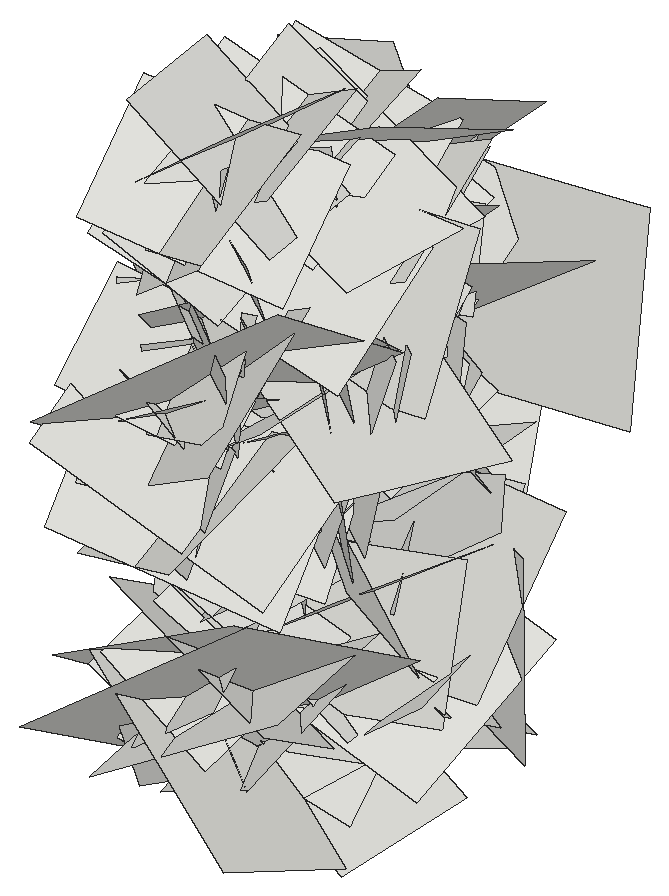
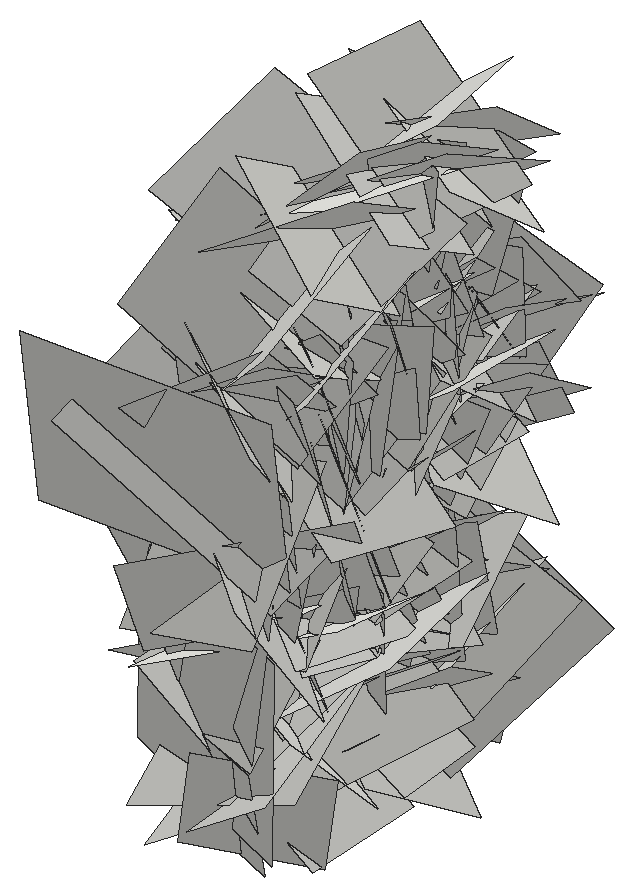
# SketchUp Ruby script. Lengths in inches.
U = 1.inch
M = Sketchup.active_model
def pt(a) = Geom::Point3d.new(a.map { |v| v * U })
def face(e, loops, mat)
  f = e.add_face(loops[0].map { |a| pt(a) })
  loops[1..].each { |l| e.add_face(l.map { |a| pt(a) }).erase! }
  f.material = f.back_material = mat if mat
  f
end
# faces: each face lists its corners as indices into pts; further lists are holes
def faces(e, pts, list, mat = nil) = list.each { |f| face(e, (f[0].is_a?(Array) ? f : [f]).map { |l| l.map { |i| pts[i] } }, mat) }
# xy, xz, yz: faces in a plane at the given z, y or x. An outline is a flat list of corners, or four numbers for a rectangle; further outlines are holes
def ring(l) = l.size == 4 ? [[l[0], l[1]], [l[2], l[1]], [l[2], l[3]], [l[0], l[3]]] : l.each_slice(2).to_a
def flat(e, list, mat, &to3) = list.each { |f| face(e, (f[0].is_a?(Array) ? f : [f]).map { |l| ring(l).map { |u, v| to3.(u, v) } }, mat) }
def xy(e, z, list, mat = nil) = flat(e, list, mat) { |x, y| [x, y, z] }
def xz(e, y, list, mat = nil) = flat(e, list, mat) { |x, z| [x, y, z] }
def yz(e, x, list, mat = nil) = flat(e, list, mat) { |y, z| [x, y, z] }
def lines(e, pts, list) = list.each { |a, b| e.add_line(pt(pts[a]), pt(pts[b])) }
# prism: a flat outline (further loops are holes) pulled along v
def prism(e, loops, v, mat = nil)
  f = face(e, loops, mat); d = Geom::Vector3d.new(v.map { |x| x * U })
  f.pushpull(f.normal.samedirection?(d) ? d.length : -d.length)
end
def box(e, o, s, mat = nil) = prism(e, [[o, [o[0] + s[0], o[1], o[2]], [o[0] + s[0], o[1] + s[1], o[2]], [o[0], o[1] + s[1], o[2]]]], [0, 0, s[2]], mat)
def at(x, y, z, deg = 0) = Geom::Transformation.translation(pt([x, y, z])) * Geom::Transformation.rotation(ORIGIN, Z_AXIS, deg.degrees)
def axes(o, x, y, z) = Geom::Transformation.new([*x, 0, *y, 0, *z, 0, *pt(o).to_a, 1])
def part(name) = M.definitions.add(name)
# library, detail: a bought-in or finely detailed component or shape, given as its bounding box
def library(name, o, s) = part(name).tap { |d| box(d.entities, o, s) }
def detail(e, o, s) = box(e.add_group.entities, o, s)
def put(e, d, t, mat = nil) = e.add_instance(d, t).tap { |i| i.material = mat if mat }
def group(e, t, mat = nil) = e.add_group.tap { |g| g.transformation = t; g.material = mat if mat }.entities
root = M.entities
c1 = part("Component\#6")
p = [[0.01,0,0],[0,3.24,4.54],[4.32,3.24,4.54],[4.33,0,0]]
faces(c1.entities,p,[[0,1,2,3]])
put(root,c1,axes([34.14,211.4,20.36],[-0.11841,0.02386,0.67628],[0.07272,0.6823,-0.01274],[0.7136,-0.06557,0.11352]))
put(root,c1,axes([34.14,208.95,27.68],[-0.1117,0.11156,-0.75397],[-0.06454,-0.75994,-0.10393],[0.80532,-0.04543,-0.11291]))
put(root,c1,axes([34.14,203.96,20.97],[0.02025,-0.24988,0.58047],[-0.03388,0.57961,0.25056],[0.66903,0.03691,-0.00488]))
put(root,c1,axes([34.14,202.42,34.22],[-0.03507,0.56649,-0.26791],[0.06705,-0.26389,-0.56581],[0.66085,0.05684,0.04319]))
put(root,c1,axes([38.11,211.47,22.62],[0.20513,-1.22241,0.07319],[0.04122,0.08019,1.23659],[-1.29742,-0.19072,0.05085]))
put(root,c1,axes([38.11,206.36,33.23],[0.09168,1.1059,0.20164],[0.04784,0.19866,-1.1089],[-1.19063,0.09314,-0.02903]))
put(root,c1,axes([38.11,205.67,24.52],[-0.15369,0.87531,0.08009],[0.01982,0.08422,-0.88666],[-0.9315,-0.14262,-0.03208]))
put(root,c1,axes([38.11,207.21,30.03],[0.00943,-1.01637,-0.0193],[0.00822,-0.01923,1.01638],[-1.07752,-0.00904,0.00758]))
put(root,c1,axes([34.14,204.95,35.05],[0.03568,0.1968,-0.61743],[-0.04358,-0.61637,-0.1987],[0.68554,-0.04943,0.01951]))
put(root,c1,axes([34.14,212.36,26.625],[-0.06935,-0.64087,-0.11796],[0.11905,-0.12787,0.63241],[0.68039,-0.04294,-0.12268]))
put(root,c1,axes([34.14,206.625,39.5],[-0.00312,0.09172,-0.66161],[0.00201,-0.66161,-0.09173],[0.70801,0.00228,-0.00265]))
put(root,c1,axes([34.14,204.22,36.67],[0.08595,0.41822,-0.43473],[-0.01861,-0.43682,-0.42351],[0.63917,-0.06896,0.04613]))
put(root,c1,axes([34.14,202.23,33.91],[0.02493,0.60398,0.49928],[-0.17768,0.49182,-0.58706],[0.81142,0.08914,-0.14389]))
put(root,c1,axes([34.14,200.85,29.625],[-0.04324,0.39016,0.69087],[-0.10275,0.68414,-0.39209],[0.83473,0.10443,-0.01247]))
put(root,c1,axes([34.14,212.78,35.18],[-0.06835,-0.19577,-0.64021],[0.13077,-0.63563,0.18195],[0.69749,0.09999,-0.09685]))
put(root,c1,axes([34.14,211.1,35.2],[0.07899,0.5337,0.27791],[0.02897,0.27674,-0.53878],[0.63716,-0.07875,-0.00996]))
put(root,c1,axes([38.11,202.75,27.49],[0.17368,0.85862,-0.51485],[-0.1903,-0.48804,-0.87105],[-1.04401,0.2318,0.07312]))
put(root,c1,axes([34.14,206.77,29.69],[0.13468,0.0618,0.68245],[-0.14259,0.68282,-0.03679],[0.71222,0.12502,-0.13642]))
put(root,c1,axes([38.11,204.74,34.65],[-0.08046,-0.48471,-0.63269],[-0.12911,-0.62103,0.49039],[-0.83492,0.14274,-0.01486]))
put(root,c1,axes([38.11,210.61,30.96],[-0.02538,-1.03384,0.49264],[0.2847,0.47394,1.00764],[-1.18007,0.13657,0.23251]))
put(root,c1,axes([38.11,212.48,33.12],[-0.02538,-1.03384,0.49264],[0.2847,0.47394,1.00764],[-1.18007,0.13657,0.23251]))
put(root,c1,axes([38.11,201.41,38.375],[0.12316,0.77538,0.57304],[-0.12545,0.58429,-0.76661],[-1.01427,0.02189,0.1644]))
put(root,c1,axes([34.14,207.11,31.75],[-0.23783,0.22127,0.93353],[-0.03566,0.95632,-0.23476],[1.01634,0.08533,0.21022]))
put(root,c1,axes([38.11,210.23,35.31],[-0.06568,0.00099,-0.81141],[-0.08224,-0.81005,0.00494],[-0.85616,0.07773,0.06177]))
put(root,c1,axes([34.14,204.33,34.72],[-0.02793,-0.28222,0.66343],[0.05268,0.66158,0.28341],[0.7624,-0.05605,0.00473]))
put(root,c1,axes([34.14,209.27,26.93],[0.01951,-0.6006,0.29742],[0.06663,0.29777,0.59742],[0.70729,-0.01148,-0.06448]))
put(root,c1,axes([38.11,205.35,34.65],[-0.12302,0.37909,0.72016],[0.00858,0.72795,-0.38188],[-0.86263,-0.04682,-0.1065]))
put(root,c1,axes([38.11,204.65,32.19],[-0.14144,0.68446,-0.34907],[-0.03425,-0.35898,-0.69154],[-0.81371,-0.10387,0.08978]))
put(root,c1,axes([34.14,205,37.54],[0.1597,-0.46751,-0.41946],[-0.05532,-0.43919,0.47075],[0.66349,0.07592,0.14021]))
put(root,c1,axes([34.14,211.91,37.97],[-0.10192,-0.72839,-0.40458],[-0.00784,-0.4065,0.73361],[0.88316,-0.08767,-0.04018]))
put(root,c1,axes([34.14,207.4,37.82],[-0.14382,-0.92009,0.02073],[-0.06912,0.03051,0.92748],[0.97309,-0.13382,0.06894]))
put(root,c1,axes([38.11,206.58,28.49],[-0.01093,-0.51913,0.63451],[-0.10311,0.63085,0.51456],[-0.86287,-0.06881,-0.06953]))
put(root,c1,axes([34.14,201.89,25.36],[0.12511,0.60489,0.30184],[-0.04372,0.31228,-0.60968],[0.71524,-0.08672,-0.09007]))
put(root,c1,axes([34.14,209.37,33.75],[-0.00852,0.3462,-0.76666],[-0.09329,-0.76284,-0.34355],[0.88678,-0.07692,-0.04351]))
put(root,c1,axes([38.11,210.92,34.25],[-0.13403,0.53039,0.57824],[0.04314,0.58935,-0.53168],[-0.83061,-0.05497,-0.12092]))
put(root,c1,axes([34.14,209.14,33.82],[0.16184,0.36707,0.52708],[-0.01835,0.54392,-0.37378],[0.68059,-0.07262,-0.13541]))
put(root,c1,axes([38.11,204.07,39.0625],[0.02986,0.79051,0.40956],[-0.00815,0.40997,-0.79076],[-0.94369,0.02147,0.01979]))
put(root,c1,axes([34.14,207.43,34.16],[0.11276,0.04323,0.70746],[-0.03845,0.71477,-0.03823],[0.75032,0.03013,-0.10828]))
put(root,c1,axes([38.11,200.125,30.08],[0.25415,0.9144,0.59243],[0.00684,0.60541,-0.93704],[-1.1549,0.20481,0.12483]))
put(root,c1,axes([38.11,209.72,22.08],[0.18138,-0.91546,-0.54155],[0.07402,-0.53767,0.93095],[-1.12504,-0.18297,-0.02606]))
put(root,c1,axes([38.11,208.86,27.22],[0.22907,0.58895,0.94038],[0.09031,0.94642,-0.61231],[-1.17269,0.18793,0.13653]))
put(root,c1,axes([38.11,209.27,26.87],[-0.02942,-0.98917,0.00062],[0.2303,-0.00549,0.9654],[-1.02292,0.02721,0.21733]))
put(root,c1,axes([34.14,202.89,32.22],[-0.0211,0.0618,0.84202],[-0.01452,0.84212,-0.06213],[0.89482,0.01512,0.01885]))
put(root,c1,axes([38.11,210.17,27.25],[-0.0389,-0.19659,0.74237],[-0.03773,0.74285,0.19496],[-0.81316,-0.02506,-0.04456]))
put(root,c1,axes([38.11,209.1,25.86],[0.06992,-0.92649,-0.30548],[0.11921,-0.29692,0.92479],[-1.02719,-0.09753,0.08653]))
put(root,c1,axes([34.14,209.1,25.86],[-0.06992,-0.92649,-0.30548],[-0.11921,-0.29692,0.92479],[1.02719,-0.09753,0.08653]))
put(root,c1,axes([34.14,210.17,27.25],[0.0389,-0.19659,0.74237],[0.03773,0.74285,0.19496],[0.81316,-0.02506,-0.04456]))
put(root,c1,axes([38.11,202.89,32.22],[0.0211,0.0618,0.84202],[0.01452,0.84212,-0.06213],[-0.89482,0.01512,0.01885]))
put(root,c1,axes([34.14,209.27,26.87],[0.02942,-0.98917,0.00062],[-0.2303,-0.00549,0.9654],[1.02292,0.02721,0.21733]))
put(root,c1,axes([34.14,208.86,27.22],[-0.22907,0.58895,0.94038],[-0.09031,0.94642,-0.61231],[1.17269,0.18793,0.13653]))
put(root,c1,axes([34.14,209.72,22.08],[-0.18138,-0.91546,-0.54155],[-0.07402,-0.53767,0.93095],[1.12504,-0.18297,-0.02606]))
put(root,c1,axes([34.14,200.125,30.08],[-0.25415,0.9144,0.59243],[-0.00684,0.60541,-0.93704],[1.1549,0.20481,0.12483]))
put(root,c1,axes([38.11,207.43,34.16],[-0.11276,0.04323,0.70746],[0.03845,0.71477,-0.03823],[-0.75032,0.03013,-0.10828]))
put(root,c1,axes([34.14,204.07,39.0625],[-0.02986,0.79051,0.40956],[0.00815,0.40997,-0.79076],[0.94369,0.02147,0.01979]))
put(root,c1,axes([38.11,209.14,33.82],[-0.16184,0.36707,0.52708],[0.01835,0.54392,-0.37378],[-0.68059,-0.07262,-0.13541]))
put(root,c1,axes([34.14,210.92,34.25],[0.13403,0.53039,0.57824],[-0.04314,0.58935,-0.53168],[0.83061,-0.05497,-0.12092]))
put(root,c1,axes([38.11,209.37,33.75],[0.00852,0.3462,-0.76666],[0.09329,-0.76284,-0.34355],[-0.88678,-0.07692,-0.04351]))
put(root,c1,axes([38.11,201.89,25.36],[-0.12511,0.60489,0.30184],[0.04372,0.31228,-0.60968],[-0.71524,-0.08672,-0.09007]))
put(root,c1,axes([34.14,206.58,28.49],[0.01093,-0.51913,0.63451],[0.10311,0.63085,0.51456],[0.86287,-0.06881,-0.06953]))
put(root,c1,axes([38.11,207.4,37.82],[0.14382,-0.92009,0.02073],[0.06912,0.03051,0.92748],[-0.97309,-0.13382,0.06894]))
put(root,c1,axes([38.11,211.91,37.97],[0.10192,-0.72839,-0.40458],[0.00784,-0.4065,0.73361],[-0.88316,-0.08767,-0.04018]))
put(root,c1,axes([38.11,205,37.54],[-0.1597,-0.46751,-0.41946],[0.05532,-0.43919,0.47075],[-0.66349,0.07592,0.14021]))
put(root,c1,axes([34.14,204.65,32.19],[0.14144,0.68446,-0.34907],[0.03425,-0.35898,-0.69154],[0.81371,-0.10387,0.08978]))
put(root,c1,axes([34.14,205.35,34.65],[0.12302,0.37909,0.72016],[-0.00858,0.72795,-0.38188],[0.86263,-0.04682,-0.1065]))
put(root,c1,axes([38.11,209.27,26.93],[-0.01951,-0.6006,0.29742],[-0.06663,0.29777,0.59742],[-0.70729,-0.01148,-0.06448]))
put(root,c1,axes([38.11,204.33,34.72],[0.02793,-0.28222,0.66343],[-0.05268,0.66158,0.28341],[-0.7624,-0.05605,0.00473]))
put(root,c1,axes([34.14,210.23,35.31],[0.06568,0.00099,-0.81141],[0.08224,-0.81005,0.00494],[0.85616,0.07773,0.06177]))
put(root,c1,axes([38.11,207.11,31.75],[0.23783,0.22127,0.93353],[0.03566,0.95632,-0.23476],[-1.01634,0.08533,0.21022]))
put(root,c1,axes([34.14,201.41,38.375],[-0.12316,0.77538,0.57304],[0.12545,0.58429,-0.76661],[1.01427,0.02189,0.1644]))
put(root,c1,axes([34.14,210.61,30.96],[0.02538,-1.03384,0.49264],[-0.2847,0.47394,1.00764],[1.18007,0.13657,0.23251]))
put(root,c1,axes([34.14,212.48,33.12],[0.02538,-1.03384,0.49264],[-0.2847,0.47394,1.00764],[1.18007,0.13657,0.23251]))
put(root,c1,axes([34.14,204.74,34.65],[0.08046,-0.48471,-0.63269],[0.12911,-0.62103,0.49039],[0.83492,0.14274,-0.01486]))
put(root,c1,axes([38.11,206.77,29.69],[-0.13468,0.0618,0.68245],[0.14259,0.68282,-0.03679],[-0.71222,0.12502,-0.13642]))
put(root,c1,axes([34.14,202.75,27.49],[-0.17368,0.85862,-0.51485],[0.1903,-0.48804,-0.87105],[1.04401,0.2318,0.07312]))
put(root,c1,axes([38.11,211.1,35.2],[-0.07899,0.5337,0.27791],[-0.02897,0.27674,-0.53878],[-0.63716,-0.07875,-0.00996]))
put(root,c1,axes([38.11,212.78,35.18],[0.06835,-0.19577,-0.64021],[-0.13077,-0.63563,0.18195],[-0.69749,0.09999,-0.09685]))
put(root,c1,axes([38.11,200.85,29.625],[0.04324,0.39016,0.69087],[0.10275,0.68414,-0.39209],[-0.83473,0.10443,-0.01247]))
put(root,c1,axes([38.11,202.23,33.91],[-0.02493,0.60398,0.49928],[0.17768,0.49182,-0.58706],[-0.81142,0.08914,-0.14389]))
put(root,c1,axes([38.11,204.22,36.67],[-0.08595,0.41822,-0.43473],[0.01861,-0.43682,-0.42351],[-0.63917,-0.06896,0.04613]))
put(root,c1,axes([38.11,206.625,39.5],[0.00312,0.09172,-0.66161],[-0.00201,-0.66161,-0.09173],[-0.70801,0.00228,-0.00265]))
put(root,c1,axes([38.11,212.36,26.625],[0.06935,-0.64087,-0.11796],[-0.11905,-0.12787,0.63241],[-0.68039,-0.04294,-0.12268]))
put(root,c1,axes([38.11,204.95,35.05],[-0.03568,0.1968,-0.61743],[0.04358,-0.61637,-0.1987],[-0.68554,-0.04943,0.01951]))
put(root,c1,axes([34.14,207.21,30.03],[-0.00943,-1.01637,-0.0193],[-0.00822,-0.01923,1.01638],[1.07752,-0.00904,0.00758]))
put(root,c1,axes([34.14,205.67,24.52],[0.15369,0.87531,0.08009],[-0.01982,0.08422,-0.88666],[0.9315,-0.14262,-0.03208]))
put(root,c1,axes([34.14,206.36,33.23],[-0.09168,1.1059,0.20164],[-0.04784,0.19866,-1.1089],[1.19063,0.09314,-0.02903]))
put(root,c1,axes([34.14,211.47,22.62],[-0.20513,-1.22241,0.07319],[-0.04122,0.08019,1.23659],[1.29742,-0.19072,0.05085]))
put(root,c1,axes([38.11,202.42,34.22],[0.03507,0.56649,-0.26791],[-0.06705,-0.26389,-0.56581],[-0.66085,0.05684,0.04319]))
put(root,c1,axes([38.11,203.96,20.97],[-0.02025,-0.24988,0.58047],[0.03388,0.57961,0.25056],[-0.66903,0.03691,-0.00488]))
put(root,c1,axes([38.11,208.95,27.68],[0.1117,0.11156,-0.75397],[0.06454,-0.75994,-0.10393],[-0.80532,-0.04543,-0.11291]))
put(root,c1,axes([38.11,211.4,20.36],[0.11841,0.02386,0.67628],[-0.07272,0.6823,-0.01274],[-0.7136,-0.06557,0.11352]))
put(root,c1,axes([34.14,209.77,25.57],[-0.04769,1.02209,-0.46416],[-0.05126,-0.46587,-1.02116],[1.18879,0.02092,-0.06265]))
put(root,c1,axes([34.14,212.41,27.7],[0.11035,-0.46639,-0.85158],[-0.0233,-0.85737,0.46687],[1.02892,0.03061,0.1019]))
put(root,c1,axes([38.11,210.37,37.54],[0.0852,-0.7988,-0.26142],[0.21653,-0.23617,0.78446],[-0.8642,-0.13792,0.17078]))
put(root,c1,axes([38.11,207.84,29.22],[0.13906,-0.51177,-0.49755],[-0.00544,-0.50655,0.51967],[-0.75658,-0.09042,-0.09518]))
put(root,c1,axes([34.14,211.63,27.44],[0.13698,0.50835,-0.7639],[0.02564,-0.77306,-0.51036],[0.97231,-0.05123,0.12108]))
put(root,c1,axes([34.14,212.85,24.81],[-0.10314,-0.72888,-0.73382],[0.20394,-0.73695,0.70648],[1.07722,0.06973,-0.20401]))
put(root,c1,axes([34.14,211.43,33.78],[-0.23599,-0.36182,-1.29322],[-0.09706,-1.30373,0.38052],[1.42014,-0.14923,-0.18889]))
put(root,c1,axes([34.14,199.54,32.72],[-0.14681,1.15124,0.44909],[-0.05729,0.44582,-1.15954],[1.30862,0.14867,-0.00039]))
put(root,c1,axes([34.14,206.07,20.81],[-0.31441,-1.20333,0.63493],[-0.01893,0.65323,1.22967],[1.44208,-0.25378,0.15457]))
put(root,c1,axes([34.14,208.01,36.375],[-0.10923,0.38133,-1.06486],[0.05778,-1.06635,-0.38714],[1.19755,0.08623,-0.07845]))
put(root,c1,axes([34.14,212.99,32.26],[0.05541,-0.21084,-0.92918],[0.15034,-0.91849,0.21639],[0.99872,0.14996,0.01898]))
put(root,c1,axes([34.14,205.46,33.43],[0.14097,0.63084,0.7943],[-0.06243,0.80455,-0.62912],[1.07339,-0.03606,-0.14091]))
put(root,c1,axes([34.14,207.91,30.98],[-0.03881,-0.77727,0.6188],[0.26695,0.59174,0.75817],[1.01873,-0.18467,-0.1751]))
put(root,c1,axes([38.11,206,31.6],[0.1462,-0.08624,0.716],[0.07336,0.72719,0.07426],[-0.76092,0.05354,0.14472]))
put(root,c1,axes([38.11,210.56,30.82],[0.08988,0.23539,0.56706],[-0.00516,0.57268,-0.23699],[-0.65079,0.02797,0.0802]))
put(root,c1,axes([34.14,206.55,33.15],[0.00164,-0.95203,-0.71322],[-0.09471,-0.7113,0.94927],[1.25737,-0.05234,0.07244]))
put(root,c1,axes([34.14,206.8125,26.89],[-0.15204,1.11982,0.24611],[0.19339,0.26716,-1.10927],[1.19986,0.09884,0.20998]))
put(root,c1,axes([34.14,211.99,33.59],[-0.13241,-0.25962,-1.28668],[-0.09489,-1.2878,0.26854],[1.38813,-0.1128,-0.10438]))
put(root,c1,axes([34.14,206.95,24.98],[0.09414,0.39654,1.07266],[-0.12922,1.07305,-0.38659],[1.20532,0.08407,-0.12522]))
put(root,c1,axes([38.11,202.49,32.61],[0.11645,-0.17214,0.59947],[0.01233,0.60916,0.17278],[-0.661,-0.01896,0.10883]))
put(root,c1,axes([34.14,205.38,23.16],[0.04798,1.09948,0.05597],[0.01409,0.05547,-1.10036],[1.16688,-0.04588,0.01099]))
put(root,c1,axes([34.14,210.75,36.02],[-0.14272,-1.0645,0.43866],[0.22696,0.41079,1.0626],[1.19913,-0.20445,-0.14891]))
put(root,c1,axes([34.14,208.81,31.45],[-0.04602,0.84125,-1.04893],[-0.18208,-1.04435,-0.83047],[1.4136,-0.10713,-0.14111]))
put(root,c1,axes([34.14,213.59,29.33],[0.10669,0.07311,-1.12569],[-0.06812,-1.12796,-0.079],[1.19381,-0.0709,0.09609]))
put(root,c1,axes([34.14,201.95,25.76],[0.02109,1.10253,-0.4508],[-0.04504,-0.44992,-1.10225],[1.2618,-0.03449,-0.03181]))
put(root,c1,axes([34.14,213.06,27.02],[-0.109,-1.16412,-0.17966],[0.1638,-0.19212,1.15639],[1.23778,-0.07709,-0.16885]))
put(root,c1,axes([34.14,201.85,37.73],[-0.10519,1.13817,0.58904],[-0.00109,0.59073,-1.14161],[1.35845,0.08861,0.0447]))
put(root,c1,axes([34.14,204.59,30.02],[-0.04301,-1.09683,0.72238],[-0.12053,0.72294,1.0913],[1.38692,0.02882,0.11724]))
put(root,c1,axes([34.14,209.74,33.23],[0.15201,0.07034,-1.21602],[-0.20156,-1.20811,-0.09231],[1.2753,-0.19933,0.13035]))
put(root,c1,axes([34.14,208.94,26.04],[-0.1299,1.02121,-0.60997],[0.25035,-0.5801,-1.01865],[1.23578,0.22487,0.14225]))
put(root,c1,axes([34.14,213.71,29.11],[-0.07729,-1.24842,0.49404],[-0.03127,0.49613,1.24937],[1.42283,-0.05691,0.0543]))
put(root,c1,axes([34.14,211.375,32.78],[-0.08242,0.8278,-0.94283],[0.12426,-0.93571,-0.83122],[1.32412,0.13934,0.01932]))
put(root,c1,axes([34.14,211.85,35.53],[0.11979,-0.95717,-0.48165],[0.13908,-0.46832,0.96146],[1.12727,0.15949,-0.06744]))
put(root,c1,axes([34.14,203.71,22.72],[-0.0324,0.32539,1.27516],[0.00551,1.27553,-0.32536],[1.39498,0.00251,0.0309]))
put(root,c1,axes([34.14,205.99,22.98],[0.14358,-1.11124,-0.06865],[0.09474,-0.05808,1.11649],[1.17635,0.14031,-0.08154]))
put(root,c1,axes([34.14,205.63,39.17],[0.17317,1.06099,0.10432],[0.22006,0.07185,-1.05594],[1.10844,-0.18002,0.19334]))
put(root,c1,axes([34.14,205.46,24.09],[0.08024,0.04196,1.34674],[-0.06239,1.34768,-0.03868],[1.42687,0.05657,-0.07742]))
put(root,c1,axes([34.14,204.65,33.57],[0.11682,0.36237,1.1463],[0.15256,1.13885,-0.37385],[1.26518,-0.17079,-0.06076]))
put(root,c1,axes([34.14,211.92,20.51],[0.20622,-1.25394,-0.15944],[-0.06822,-0.17093,1.26581],[1.33814,0.18453,0.0891]))
put(root,c1,axes([34.14,213.57,27.56],[-0.01798,0.03957,-1.39555],[0.22262,-1.3797,-0.04168],[1.46303,0.21042,-0.01081]))
put(root,c1,axes([34.14,205.51,24.88],[0.13882,1.11155,0.63897],[0.19603,0.6192,-1.11507],[1.34484,-0.205,0.09658]))
put(root,c1,axes([33.8,214.11,35.21],[0.07772,-0.27644,-1.33377],[0.91911,-1.02064,0.2592],[1.11351,0.86175,-0.12086]))
put(root,c1,axes([34.14,205.05,35.75],[0.23328,1.34713,-0.22992],[0.05022,-0.24027,-1.36238],[1.44774,-0.20874,0.08431]))
put(root,c1,axes([34.14,206.12,25.83],[0.28838,0.48251,1.20317],[0.13396,1.21365,-0.51529],[1.36755,-0.22063,-0.20324]))
